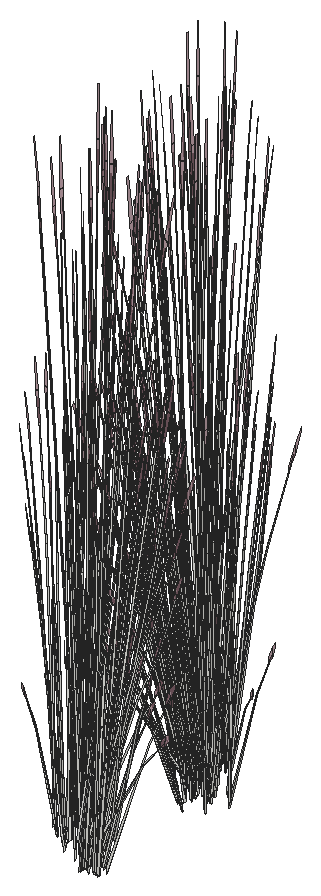
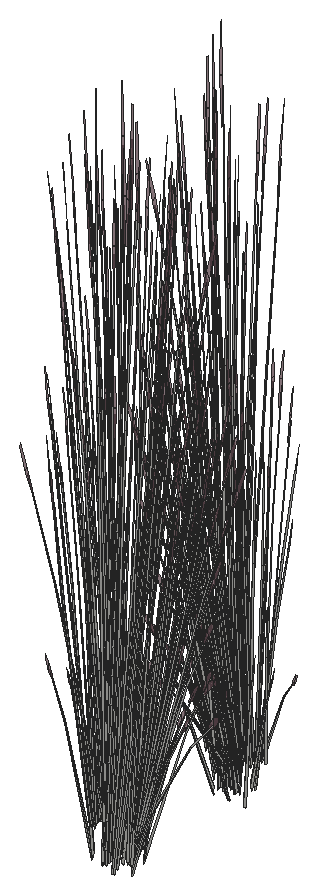
# SketchUp Ruby script. Lengths in inches.
U = 1.inch
M = Sketchup.active_model
def pt(a) = Geom::Point3d.new(a.map { |v| v * U })
def face(e, loops, mat)
  f = e.add_face(loops[0].map { |a| pt(a) })
  loops[1..].each { |l| e.add_face(l.map { |a| pt(a) }).erase! }
  f.material = f.back_material = mat if mat
  f
end
# faces: each face lists its corners as indices into pts; further lists are holes
def faces(e, pts, list, mat = nil) = list.each { |f| face(e, (f[0].is_a?(Array) ? f : [f]).map { |l| l.map { |i| pts[i] } }, mat) }
# xy, xz, yz: faces in a plane at the given z, y or x. An outline is a flat list of corners, or four numbers for a rectangle; further outlines are holes
def ring(l) = l.size == 4 ? [[l[0], l[1]], [l[2], l[1]], [l[2], l[3]], [l[0], l[3]]] : l.each_slice(2).to_a
def flat(e, list, mat, &to3) = list.each { |f| face(e, (f[0].is_a?(Array) ? f : [f]).map { |l| ring(l).map { |u, v| to3.(u, v) } }, mat) }
def xy(e, z, list, mat = nil) = flat(e, list, mat) { |x, y| [x, y, z] }
def xz(e, y, list, mat = nil) = flat(e, list, mat) { |x, z| [x, y, z] }
def yz(e, x, list, mat = nil) = flat(e, list, mat) { |y, z| [x, y, z] }
def lines(e, pts, list) = list.each { |a, b| e.add_line(pt(pts[a]), pt(pts[b])) }
# prism: a flat outline (further loops are holes) pulled along v
def prism(e, loops, v, mat = nil)
  f = face(e, loops, mat); d = Geom::Vector3d.new(v.map { |x| x * U })
  f.pushpull(f.normal.samedirection?(d) ? d.length : -d.length)
end
def box(e, o, s, mat = nil) = prism(e, [[o, [o[0] + s[0], o[1], o[2]], [o[0] + s[0], o[1] + s[1], o[2]], [o[0], o[1] + s[1], o[2]]]], [0, 0, s[2]], mat)
def at(x, y, z, deg = 0) = Geom::Transformation.translation(pt([x, y, z])) * Geom::Transformation.rotation(ORIGIN, Z_AXIS, deg.degrees)
def axes(o, x, y, z) = Geom::Transformation.new([*x, 0, *y, 0, *z, 0, *pt(o).to_a, 1])
def part(name) = M.definitions.add(name)
# library, detail: a bought-in or finely detailed component or shape, given as its bounding box
def library(name, o, s) = part(name).tap { |d| box(d.entities, o, s) }
def detail(e, o, s) = box(e.add_group.entities, o, s)
def put(e, d, t, mat = nil) = e.add_instance(d, t).tap { |i| i.material = mat if mat }
def group(e, t, mat = nil) = e.add_group.tap { |g| g.transformation = t; g.material = mat if mat }.entities
root = M.entities
M.materials.add("LightPink_Translucent").color = [144, 107, 117]
M.materials["LightPink_Translucent"].alpha = 0.75
c1 = part("blade")
p = [[2.15,0.21,22],[0,0.17,0],[0.09,0.45,0],[2.18,0.31,22],[2.29,0.31,22],[0.38,0.45,0],
  [2.48,0.24,33],[2.49,0.24,33],[2.48,0.22,33]]
faces(c1.entities,p,[[0,1,2,3],[4,5,2,3],[6,3,4,7],[8,0,3,6]])
c2 = part("seeds")
p = [[0.3,-0.1,1.38],[-0.01,-0.03,1.59],[-0.01,-0.03,0.03],[0.14,-0.07,-0.07],[0.29,-0.03,3],[0.15,0.01,3.11]]
faces(c2.entities,p,[[0,1,2,3],[1,0,4,5]],"LightPink_Translucent")
c3 = part("blade with seeds")
put(c3.entities,c1,at(0,0,0))
put(c3.entities,c2,axes([2.4,0.25,30.99],[1.5799,-0.05474,1.17369],[-0.12525,1.92788,0.29478],[-0.07173,-0.02425,1.56792]))
put(root,c3,axes([330.45,409.64,1400.48],[0.33032,0.23318,0.49651],[-0.19744,0.41812,0],[-0.07523,-0.05311,1.57504]))
put(root,c3,axes([331.62,408.02,1400.72],[0.17124,-0.42022,0.44739],[0.35581,0.20224,-0.21531],[0,0.09687,1.43643]))
put(root,c3,axes([333.3,409.9,1402.71],[-0.03191,-0.04083,1.77383],[0.06981,-0.43764,-0.16761],[0.12571,-0.02796,0.31391]))
put(root,c3,axes([329.14,408.125,1402.72],[-0.05763,0.06055,1.74944],[0.0049,0.44239,-0.27667],[-0.13211,0.05753,0.14031]))
put(root,c3,axes([331.55,408.26,1400.29],[0,0.53934,-0.05637],[-0.44133,0,0],[0,0.01695,1.79368]))
put(root,c3,axes([329.53,408.07,1402.68],[-0.09562,0.42421,-0.51099],[-0.32782,-0.1454,-0.3958],[-0.13199,0.0389,0.97773]))
put(root,c3,axes([329.51,407.71,1403.03],[0.17758,0.42229,-0.1216],[-0.31518,0.20752,-0.67495],[-0.13282,0.05572,1.02557]))
put(root,c3,axes([331.58,407.88,1400.21],[0.21202,0.39143,-0.44739],[-0.32115,0.27564,0.21531],[0.06861,0.04843,1.43643]))
put(root,c3,axes([333.02,409.54,1401.93],[-0.06755,-0.39203,-0.03492],[0.31928,-0.09013,-0.15832],[0.06667,0.02485,0.52218]))
put(root,c3,axes([330.26,409.88,1400.375],[-0.22066,0.46731,0],[-0.36918,-0.26061,-0.51607],[-0.08408,-0.05936,1.63711]))
put(root,c3,axes([332.19,409.53,1403.03],[0.0189,-0.47427,-0.1216],[0.35781,0.01296,-0.67495],[0.13781,0.03295,1.02557]))
put(root,c3,axes([332.52,408.26,1400.48],[0,-0.46636,0.49651],[0.39487,0,0],[0,0.10622,1.57504]))
put(root,c3,axes([331.53,408.61,1400.72],[0.38326,-0.02879,0.44739],[0.03466,0.47788,-0.21531],[-0.06861,0.04843,1.43643]))
put(root,c3,axes([331.77,408.12,1400.62],[0.32884,-0.136,0.1448],[0.11516,0.38837,-0.41347],[0,0.08547,1.26744]))
put(root,c3,axes([332.14,409.34,1403.05],[-0.20082,-0.29199,0.35414],[0.2293,-0.2764,-0.4572],[0.1165,0.04206,0.87481]))
put(root,c3,axes([331.1875,408.84,1400.21],[-0.38326,0.02879,-0.44739],[-0.03466,-0.47788,0.21531],[-0.06861,0.04843,1.43643]))
put(root,c3,axes([332.99,409.07,1400.59],[-0.085,-0.1147,1.43002],[0.1106,-0.37943,-0.30754],[0.17198,0.0514,0.61141]))
put(root,c3,axes([331.47,409.48,1400.2],[0.35581,0.20937,0],[-0.17124,0.43505,0],[0,0,1.74954]))
put(root,c3,axes([332.5,409.24,1402.72],[0.07571,-0.00789,1.74944],[0.20767,-0.36231,-0.27667],[0.13467,0.04783,0.14031]))
put(root,c3,axes([331.61,409.95,1400.19],[-0.21791,-0.46895,-0.05142],[0.36918,-0.26061,0.51607],[-0.09097,0.04465,1.6363]))
put(root,c3,axes([331.53,408.8125,1400.62],[0.26075,0.2802,0.1448],[-0.2175,0.31612,-0.41347],[-0.06054,0.04274,1.26744]))
put(root,c3,axes([329.47,408.89,1402.73],[-0.08753,-0.42921,0.48003],[0.34336,-0.07449,0.3958],[-0.1012,0.10094,0.9933]))
put(root,c3,axes([329.41,408.8,1402.73],[-0.2423,-0.19613,0.0643],[0.14107,-0.2793,0.50621],[-0.07768,0.0903,0.77189]))
put(root,c3,axes([329.52,408.29,1401.875],[0.12246,-0.09864,1.71376],[0.1031,0.45582,0.13857],[-0.19225,0.10302,0.73262]))
put(root,c3,axes([332.21,409.3,1402.98],[0.35281,0.01123,-0.71045],[-0.0237,0.47284,0.08574],[0.14947,0.0499,1.00501]))
put(root,c3,axes([331.8125,409.68,1400.48],[0.33032,-0.23318,0.49651],[0.19744,0.41812,0],[-0.07523,0.05311,1.57504]))
put(root,c3,axes([331.34,409.31,1400.29],[0.15345,0.53576,-0.06012],[-0.43845,0.18773,0],[0.00536,0.01871,1.72173]))
put(root,c3,axes([331.51,409.89,1400.03],[-0.32928,-0.11539,-0.30978],[0.08291,-0.40636,0.30978],[-0.06638,0.04686,1.38974]))
put(root,c3,axes([329.14,409.0625,1400.59],[0.12266,0.03828,1.43002],[0.07906,0.39104,-0.30754],[-0.16661,0.0732,0.61141]))
put(root,c3,axes([329.6875,408.74,1403.05],[0.30722,-0.06665,0.35414],[0.08112,0.381,-0.4572],[-0.08804,0.10234,0.87481]))
put(root,c3,axes([332.78,408.34,1400.375],[0.44133,0,0],[0,0.52122,-0.51607],[0,0.11871,1.63711]))
put(root,c3,axes([328.5,408.57,1402.71],[0.04504,0.01251,1.77383],[0.13934,0.41205,-0.16761],[-0.0922,0.10815,0.31391]))
put(root,c3,axes([332.61,408.61,1400.2],[-0.44111,-0.00373,-0.04976],[0,-0.52122,0.49943],[-0.01386,0.11865,1.58352]))
put(root,c3,axes([331.65,408.15,1400.67],[0.39748,0.22252,-0.29095],[-0.19139,0.46966,-0.50002],[0.01249,0.11531,1.59708]))
put(root,c3,axes([328.88,409.88,1400.77],[0.14709,-0.21136,1.1486],[0.05804,0.3346,0.84392],[-0.1063,0.05991,0.25299]))
put(root,c3,axes([332.42,409.49,1402.53],[0.20082,0.29199,-0.35414],[-0.2293,0.2764,0.4572],[0.1165,0.04206,0.87481]))
put(root,c3,axes([332.52,408.68,1400.03],[-0.24637,0.29097,-0.30978],[-0.24637,-0.29097,0.30978],[0,0.09372,1.38974]))
put(root,c3,axes([331.46,408.71,1400.67],[0.04113,0.53214,-0.29095],[-0.42835,0.03218,-0.50002],[-0.07543,0.07088,1.59708]))
put(root,c3,axes([332.32,409.6,1402.73],[-0.01777,0.35463,0.0643],[-0.26836,-0.00972,0.50621],[0.1028,0.03711,0.77189]))
put(root,c3,axes([331.61,408.5,1400.21],[-0.17124,0.42022,-0.44739],[-0.35581,-0.20224,0.21531],[0,0.09687,1.43643]))
put(root,c3,axes([329.43,408.97,1402.53],[-0.30722,0.06665,-0.35414],[-0.08112,-0.381,0.4572],[-0.08804,0.10234,0.87481]))
put(root,c3,axes([332.34,409.49,1402.73],[-0.26024,0.30729,0.48003],[-0.22444,-0.32634,0.3958],[0.1221,0.05668,0.9933]))
put(root,c3,axes([328.99,409.83,1403.65],[0.31145,0.12449,-0.06488],[-0.0958,0.38314,-0.29416],[-0.05094,0.05817,0.97024]))
put(root,c3,axes([331.2,409.12,1400.06],[-0.23773,0.35053,-0.62353],[-0.29532,-0.31785,-0.16365],[-0.09526,0.08744,1.37633]))
put(root,c3,axes([331.52,409.85,1403.05],[-0.05451,-0.37564,0.35414],[0.31161,-0.09919,-0.4572],[0.0837,0.10765,0.87481]))
put(root,c3,axes([331.62,409.71,1400.33],[0.44186,0.15158,0.30756],[-0.11054,0.54181,-0.36492],[-0.07313,0.06781,1.64885]))
put(root,c3,axes([331.59,410.07,1400.02],[-0.33032,0.23318,-0.49651],[-0.19744,-0.41812,0],[-0.07523,0.05311,1.57504]))
put(root,c3,axes([332.6875,408.69,1400.02],[0,0.46636,-0.49651],[-0.39487,0,0],[0,0.10622,1.57504]))
put(root,c3,axes([331.7,408.74,1401.875],[-0.1311,-0.08035,1.71376],[0.27131,-0.33708,0.13857],[0.16909,0.15206,0.73262]))
put(root,c3,axes([331.72,407.6875,1402.47],[-0.30498,-0.24231,1.38283],[0.32203,-0.37727,0.59665],[0.0984,0.22736,1.33663]))
put(root,c3,axes([329.53,408.71,1403.03],[0.32648,0.25715,-0.1216],[-0.18809,0.3724,-0.67495],[-0.09224,0.12945,1.02557]))
put(root,c3,axes([332.18,409.66,1400.77],[-0.19872,-0.13409,1.1486],[0.2566,-0.13625,0.84392],[0.06921,0.11541,0.25299]))
put(root,c3,axes([331.49,410.04,1403.03],[0.21031,-0.39918,-0.1216],[0.30457,0.22997,-0.67495],[0.10587,0.11278,1.02557]))
put(root,c3,axes([329.97,408.59,1401.875],[0.08815,-0.14329,1.71376],[0.22258,0.38678,0.13857],[-0.15267,0.17614,0.73262]))
put(root,c3,axes([329.6875,409.01,1402.68],[0.09067,0.42583,-0.51099],[-0.34336,0.07449,-0.3958],[-0.0984,0.11438,0.97773]))
put(root,c3,axes([330.1,409.5,1403.05],[0.23881,-0.24554,0.35414],[0.22606,0.28036,-0.4572],[-0.0344,0.14245,0.87481]))
put(root,c3,axes([331.89,410,1400.375],[0.22066,0.46731,0],[-0.36918,0.26061,-0.51607],[-0.08408,0.05936,1.63711]))
put(root,c3,axes([331.21,410.37,1402.71],[0.00104,-0.05646,1.77383],[0.30246,-0.2491,-0.16761],[0.10506,0.08891,0.31391]))
put(root,c3,axes([332.24,410.16,1399.49],[0.02571,-0.06733,1.76342],[0.32373,-0.19829,-0.26939],[0.09815,0.10263,0.30037]))
put(root,c3,axes([331.7,408.15,1400.84],[-0.00964,-0.43909,1.41272],[0.43635,0.11382,0.59816],[-0.1032,0.24027,1.3335]))
put(root,c3,axes([331.8125,408.63,1400.09],[0.12941,0.42699,-0.69212],[-0.37279,0.15378,-0.18165],[0.0143,0.14459,1.52773]))
put(root,c3,axes([329.88,409.73,1402.73],[-0.29004,-0.02173,0.0643],[0.00795,-0.32812,0.50621],[-0.03035,0.12569,0.77189]))
put(root,c3,axes([329.27,410.1,1399.49],[0.04734,0.04659,1.76342],[0.08027,0.4317,-0.26939],[-0.10492,0.09206,0.30037]))
put(root,c3,axes([329.98,409.76,1402.73],[-0.25132,-0.3182,0.48003],[0.2669,-0.27442,0.3958],[-0.04636,0.14929,0.9933]))
put(root,c3,axes([331.74,409.84,1402.68],[0.34827,-0.11086,-0.51099],[0.06092,0.41983,-0.3958],[0.09354,0.12031,0.97773]))
put(root,c3,axes([330.77,409.91,1403.05],[0.1064,-0.35863,0.35414],[0.31043,0.1046,-0.4572],[0.02846,0.14439,0.87481]))
put(root,c3,axes([332.22,410.27,1400.67],[-0.22633,-0.01463,1.0506],[0.14947,-0.31064,0.58006],[0.08941,0.11036,0.8241]))
put(root,c3,axes([331.56,410.1875,1402.73],[-0.16041,0.29625,0.0643],[-0.22843,-0.17248,0.50621],[0.07385,0.09498,0.77189]))
put(root,c3,axes([331.1875,411.1875,1403.65],[0.2439,-0.26754,-0.06488],[0.22348,0.29302,-0.29416],[0.01573,0.08303,0.97024]))
put(root,c3,axes([331.63,410.1,1402.73],[-0.35104,0.10702,0.48003],[-0.06092,-0.41983,0.3958],[0.08256,0.12373,0.9933]))
put(root,c3,axes([329.9,408.95,1401.875],[0.06572,-0.16029,1.71376],[0.27569,0.33172,0.13857],[-0.12437,0.20675,0.73262]))
put(root,c3,axes([331.48,409.52,1400.59],[0.00623,-0.15459,1.43002],[0.29764,-0.17268,-0.30754],[0.09188,0.18503,0.61141]))
put(root,c3,axes([330.67,410.23,1402.73],[-0.26007,0.1585,0.0643],[-0.12729,-0.28902,0.50621],[0.02512,0.1274,0.77189]))
put(root,c3,axes([329.98,409.85,1402.53],[-0.23881,0.24554,-0.35414],[-0.22606,-0.28036,0.4572],[-0.0344,0.14245,0.87481]))
put(root,c3,axes([329.15,409.78,1402.72],[-0.00877,0.09229,1.74944],[0.24897,0.32105,-0.27667],[-0.06518,0.15182,0.14031]))
put(root,c3,axes([329.95,409.57,1403.4],[0.3879,0.02311,-0.13498],[-0.0106,0.43749,-0.74919],[-0.02694,0.1685,1.13838]))
put(root,c3,axes([330.67,410.06,1403.03],[0.34538,-0.21713,-0.1216],[0.16972,0.38536,-0.67495],[0.04557,0.16239,1.02557]))
put(root,c3,axes([330.77,410.2,1403.0625],[-0.34777,-0.12192,0.53283],[0.11892,-0.40083,0.43934],[0.0209,0.15763,1.10256]))
put(root,c3,axes([330.13,410.8,1400.77],[-0.00913,-0.2773,1.1486],[0.22824,0.19778,0.84392],[-0.04489,0.13217,0.25299]))
put(root,c3,axes([330.73,410.14,1399.49],[0.05712,-0.02538,1.76342],[0.34359,0.13968,-0.26939],[0.01005,0.15742,0.30037]))
put(root,c3,axes([330.21,409.73,1403],[0.25266,0.31335,-0.5672],[-0.2669,0.27442,-0.43934],[-0.03844,0.15921,1.08528]))
put(root,c3,axes([329.9375,410.21,1400.82],[0.32063,-0.08258,0.06507],[0.07371,0.33271,-0.86304],[-0.02033,0.16842,0.7736]))
put(root,c3,axes([330.96,410.04,1402.68],[0.34695,0.11691,-0.51099],[-0.11892,0.40083,-0.3958],[0.03181,0.16138,0.97773]))
put(root,c3,axes([331.16,409.21,1401.875],[-0.08068,-0.14973,1.71376],[0.3728,-0.12606,0.13857],[0.08426,0.23506,0.73262]))
put(root,c3,axes([330.8,410.28,1402.53],[-0.1064,0.35863,-0.35414],[-0.31043,-0.1046,0.4572],[0.02846,0.14439,0.87481]))
put(root,c3,axes([330.13,409.59,1403.34],[-0.00918,0.43138,-0.7886],[-0.38672,-0.02897,0.09517],[-0.04081,0.18275,1.11556]))
put(root,c3,axes([329.125,410.72,1402.71],[0.04004,-0.02816,1.77383],[0.33095,0.18728,-0.16761],[-0.00778,0.15594,0.31391]))
put(root,c3,axes([330.5,409.29,1401.875],[-0.00864,-0.17899,1.71376],[0.37441,0.11874,0.13857],[-0.02316,0.25508,0.73262]))
put(root,c3,axes([330.84,409.96,1402.98],[0.16845,0.3792,-0.71045],[-0.34676,0.21133,0.08574],[0.03939,0.18322,1.00501]))
put(root,c3,axes([329.86,410.56,1400.59],[0.11138,-0.07357,1.43002],[0.27499,0.22183,-0.30754],[-0.08185,0.19194,0.61141]))
put(root,c3,axes([330.58,410.92,1402.72],[0.04474,0.0751,1.74944],[0.36104,0.0295,-0.27667],[0.03631,0.16562,0.14031]))
put(root,c3,axes([330.01,410.2,1401.36],[0.00775,-0.24075,1.54345],[0.34877,0.12716,0.21329],[-0.03022,0.25658,0.72882]))
put(root,c3,axes([330.27,421.53,1401.875],[0.08068,0.14973,1.71376],[-0.3728,0.12606,0.13857],[-0.08426,-0.23506,0.73262]))
put(root,c3,axes([330.89,420.54,1402.72],[-0.05398,-0.06539,1.74944],[-0.36026,0.04145,-0.27667],[-0.0575,-0.15639,0.14031]))
put(root,c3,axes([331.72,421.32,1400.59],[-0.10032,0.0944,1.43002],[-0.30046,-0.16522,-0.30754],[0.05569,-0.20547,0.61141]))
put(root,c3,axes([331.27,421.64,1402.98],[-0.16845,-0.3792,-0.71045],[0.34676,-0.21133,0.08574],[-0.03939,-0.18322,1.00501]))
put(root,c3,axes([330.17,421.14,1400.59],[-0.02137,0.15256,1.43002],[-0.31245,0.12771,-0.30754],[-0.07303,-0.19719,0.61141]))
put(root,c3,axes([330.98,420.8,1399.49],[-0.0592,0.0168,1.76342],[-0.32738,-0.18913,-0.26939],[0.00549,-0.15776,0.30037]))
put(root,c3,axes([331.97,422.01,1402.98],[0.00918,-0.43138,-0.71045],[0.38672,0.02897,0.08574],[0.04081,-0.18275,1.00501]))
put(root,c3,axes([332.51,421.34,1402.72],[-0.00341,-0.09282,1.74944],[-0.28775,-0.26825,-0.27667],[0.04449,-0.16261,0.14031]))
put(root,c3,axes([331.3,421.32,1402.53],[0.1064,-0.35863,-0.35414],[0.31043,0.1046,0.4572],[-0.02846,-0.14439,0.87481]))
put(root,c3,axes([331.53,421.8,1401.875],[-0.06572,0.16029,1.71376],[-0.27569,-0.33172,0.13857],[0.12437,-0.20675,0.73262]))
put(root,c3,axes([332.43,421.01,1402.71],[-0.03584,0.03562,1.77383],[-0.35118,-0.12018,-0.16761],[-0.01271,-0.15545,0.31391]))
put(root,c3,axes([331.14,421.57,1402.68],[-0.34695,-0.11691,-0.51099],[0.11892,-0.40083,-0.3958],[-0.03181,-0.16138,0.97773]))
put(root,c3,axes([331.35,420.5625,1400.77],[0.04528,0.27194,1.1486],[-0.25117,-0.15062,0.84392],[0.02703,-0.13924,0.25299]))
put(root,c3,axes([331.89,421.87,1402.68],[-0.25266,-0.31335,-0.51099],[0.2669,-0.27442,-0.3958],[0.03844,-0.15921,0.97773]))
put(root,c3,axes([330.52,420.33,1402.71],[-0.00658,0.0559,1.77383],[-0.32474,0.20287,-0.16761],[-0.09556,-0.1037,0.31391]))
put(root,c3,axes([330.45,421.32,1403.09],[0.39316,-0.11987,0.53763],[0.06823,0.47021,0.4433],[-0.09247,-0.13858,1.11249]))
put(root,c3,axes([331.34,421.4,1402.73],[0.34777,0.12192,0.48003],[-0.11892,0.40083,0.3958],[-0.0209,-0.15763,0.9933]))
put(root,c3,axes([331.4375,421.55,1403.03],[-0.34538,0.21713,-0.1216],[-0.16972,-0.38536,-0.67495],[-0.04557,-0.16239,1.02557]))
put(root,c3,axes([332.15,422.04,1403.03],[-0.3879,-0.02311,-0.1216],[0.0106,-0.43749,-0.67495],[0.02694,-0.1685,1.02557]))
put(root,c3,axes([332.13,421.76,1402.53],[0.23881,-0.24554,-0.35414],[0.22606,0.28036,0.4572],[0.0344,-0.14245,0.87481]))
put(root,c3,axes([330.0625,420.89,1400.77],[0.18411,0.16231,1.1486],[-0.26813,0.09757,0.84392],[-0.05737,-0.12474,0.25299]))
put(root,c3,axes([331.43,421.375,1402.73],[0.26007,-0.1585,0.0643],[0.12729,0.28902,0.50621],[-0.02512,-0.1274,0.77189]))
put(root,c3,axes([330.51,421.75,1402.98],[-0.30095,-0.22541,-0.71045],[0.21388,-0.395,0.08574],[-0.10904,-0.13459,1.00501]))
put(root,c3,axes([330.4,421.45,1402.53],[-0.05451,-0.37564,-0.35414],[0.31161,-0.09919,0.4572],[-0.0837,-0.10765,0.87481]))
put(root,c3,axes([330.54,421.42,1402.73],[0.16041,-0.29625,0.0643],[0.22843,0.17248,0.50621],[-0.07385,-0.09498,0.77189]))
put(root,c3,axes([329.92,421.38,1399.49],[-0.03419,0.06144,1.76342],[-0.3455,0.13246,-0.26939],[-0.08346,-0.12049,0.30037]))
put(root,c3,axes([330.49,423.07,1400.1],[-0.14494,-0.47823,-0.69835],[0.41752,-0.17223,-0.18329],[-0.01602,-0.16194,1.54149]))
put(root,c3,axes([329.73,422,1401.875],[0.1311,0.08035,1.71376],[-0.27131,0.33708,0.13857],[-0.16909,-0.15206,0.73262]))
put(root,c3,axes([332.43,421.61,1399.49],[-0.05283,-0.03674,1.76342],[-0.13569,-0.41045,-0.26939],[0.09154,-0.11138,0.30037]))
put(root,c3,axes([331.33,421.7,1403.05],[-0.1064,0.35863,0.35414],[-0.31043,-0.1046,-0.4572],[-0.02846,-0.14439,0.87481]))
put(root,c3,axes([330.37,421.76,1402.68],[-0.34827,0.11086,-0.51099],[-0.06092,-0.41983,-0.3958],[-0.09354,-0.12031,0.97773]))
put(root,c3,axes([332.125,421.85,1402.73],[0.25132,0.3182,0.48003],[-0.2669,0.27442,0.3958],[0.04636,-0.14929,0.9933]))
put(root,c3,axes([330.61,421.39,1403.43],[-0.23555,0.44708,-0.13619],[-0.34112,-0.25757,-0.75594],[-0.11858,-0.12631,1.14864]))
put(root,c3,axes([332.22,421.88,1402.73],[0.29004,0.02173,0.0643],[-0.00795,0.32812,0.50621],[0.03035,-0.12569,0.77189]))
put(root,c3,axes([332,422.1,1403.05],[-0.23881,0.24554,0.35414],[-0.22606,-0.28036,-0.4572],[0.0344,-0.14245,0.87481]))
put(root,c3,axes([332.42,422.76,1402.98],[0.18436,-0.36797,-0.71045],[0.32306,0.26151,0.08574],[0.11008,-0.13332,1.00501]))
put(root,c3,axes([330.43,421.69,1400.375],[-0.22066,-0.46731,0],[0.36918,-0.26061,-0.51607],[0.08408,-0.05936,1.63711]))
put(root,c3,axes([332.41,422.59,1402.68],[-0.09067,-0.42583,-0.51099],[0.34336,-0.07449,-0.3958],[0.0984,-0.11438,0.97773]))
put(root,c3,axes([330.92,421.13,1400.13],[-0.2439,0.26754,-0.03893],[-0.22348,-0.29302,-0.17649],[-0.01573,-0.08303,0.58215]))
put(root,c3,axes([329.71,421.26,1402.72],[-0.07594,-0.00329,1.74944],[-0.24177,0.32918,-0.27667],[-0.129,-0.06726,0.14031]))
put(root,c3,axes([332.58,422.9,1403.03],[-0.32648,-0.25715,-0.1216],[0.18809,-0.3724,-0.67495],[0.09224,-0.12945,1.02557]))
put(root,c3,axes([331.23,424.3,1401.33],[0.305,0.18805,1.51261],[-0.29879,0.40513,0.59816],[-0.13384,-0.24012,1.26806]))
put(root,c3,axes([330.59,421.76,1403.05],[0.05451,0.37564,0.35414],[-0.31161,0.09919,-0.4572],[-0.0837,-0.10765,0.87481]))
put(root,c3,axes([329.63,423,1400.02],[0,-0.46636,-0.49651],[0.39487,0,0],[0,-0.10622,1.57504]))
put(root,c3,axes([330.73,421.62,1400.02],[0.33032,-0.23318,-0.49651],[0.19744,0.41812,0],[0.07523,-0.05311,1.57504]))
put(root,c3,axes([332.69,422.43,1400.59],[-0.12609,-0.01381,1.43002],[-0.12917,-0.37055,-0.30754],[0.1549,-0.10482,0.61141]))
put(root,c3,axes([329.65,422,1403.09],[0.29147,-0.34417,0.53763],[0.25138,0.3655,0.4433],[-0.13675,-0.06349,1.11249]))
put(root,c3,axes([333.38,422.79,1402.71],[-0.0461,-0.00354,1.77383],[-0.19143,-0.37951,-0.16761],[0.07688,-0.12478,0.31391]))
put(root,c3,axes([331.12,422.58,1400.06],[0.23773,-0.35053,-0.62353],[0.29532,0.31785,-0.16365],[0.09526,-0.08744,1.37633]))
put(root,c3,axes([332.84,421.75,1400.77],[-0.11756,0.2374,1.1486],[-0.10105,-0.31895,0.84392],[0.09709,-0.07992,0.25299]))
put(root,c3,axes([332.67,422.64,1402.53],[0.30722,-0.06665,-0.35414],[0.08112,0.381,0.4572],[0.08804,-0.10234,0.87481]))
put(root,c3,axes([329.78,422,1402.73],[0.01777,-0.35463,0.0643],[0.26836,0.00972,0.50621],[-0.1028,-0.03711,0.77189]))
put(root,c3,axes([330.71,423.19,1400.21],[0.17124,-0.42022,-0.44739],[0.35581,0.20224,0.21531],[0,-0.09687,1.43643]))
put(root,c3,axes([329.68,422.11,1402.53],[-0.20082,-0.29199,-0.35414],[0.2293,-0.2764,0.4572],[-0.1165,-0.04206,0.87481]))
put(root,c3,axes([330.86,422.98,1400.67],[-0.04113,-0.53214,-0.29095],[0.42835,-0.03218,-0.50002],[0.07543,-0.07088,1.59708]))
put(root,c3,axes([329.8,423.01,1400.03],[0.24637,-0.29097,-0.30978],[0.24637,0.29097,0.30978],[0,-0.09372,1.38974]))
put(root,c3,axes([329.7,421.62,1400.13],[-0.10181,0.3808,-0.03893],[-0.31336,-0.11714,-0.17649],[-0.04758,-0.06228,0.58215]))
put(root,c3,axes([332.42,422.86,1403.05],[-0.30722,0.06665,0.35414],[-0.08112,-0.381,-0.4572],[0.08804,-0.10234,0.87481]))
put(root,c3,axes([330.67,423.54,1400.67],[-0.39748,-0.22252,-0.29095],[0.19139,-0.46966,-0.50002],[-0.01249,-0.11531,1.59708]))
put(root,c3,axes([329.53,423.36,1400.375],[-0.44133,0,0],[0,-0.52122,-0.51607],[0,-0.11871,1.63711]))
put(root,c3,axes([329.61,422.42,1400.59],[0.06891,0.12984,1.43002],[-0.15879,0.35293,-0.30754],[-0.16304,-0.08436,0.61141]))
put(root,c3,axes([330.81,421.81,1400.03],[0.32928,0.11539,-0.30978],[-0.08291,0.40636,0.30978],[0.06638,-0.04686,1.38974]))
put(root,c3,axes([329.89,422.31,1402.98],[-0.35281,-0.01123,-0.71045],[0.0237,-0.47284,0.08574],[-0.14947,-0.0499,1.00501]))
put(root,c3,axes([332.7,422.8,1402.73],[0.2423,0.19613,0.0643],[-0.14107,0.2793,0.50621],[0.07768,-0.0903,0.77189]))
put(root,c3,axes([332.63,422.72,1402.73],[0.08753,0.42921,0.48003],[-0.34336,0.07449,0.3958],[0.1012,-0.10094,0.9933]))
put(root,c3,axes([333.55,423.24,1402.72],[0.04898,-0.07104,1.74944],[-0.06269,-0.43574,-0.27667],[0.12289,-0.08262,0.14031]))
put(root,c3,axes([329.875,423.22,1400.33],[-0.32829,0.39208,0.30756],[-0.32849,-0.38796,-0.36492],[-0.01146,-0.11134,1.64885]))
put(root,c3,axes([329.42,421.54,1402.71],[0.02617,0.04654,1.77383],[-0.12614,0.41836,-0.16761],[-0.12775,0.00303,0.31391]))
put(root,c3,axes([330.92,423.4,1400.43],[0.39767,0.22603,0.24065],[-0.19139,0.46966,0.50002],[0,-0.10827,1.60543]))
put(root,c3,axes([330.77,424.04,1400.4375],[0.09355,-0.55261,-0.23429],[0.44354,0.09633,0.51271],[-0.0775,-0.07631,1.5644]))
put(root,c3,axes([329.78,422.4,1402.68],[-0.25628,0.30892,-0.51099],[-0.22444,-0.32634,-0.3958],[-0.13021,-0.047,0.97773]))
put(root,c3,axes([329.97,422.27,1403.05],[0.20082,0.29199,0.35414],[-0.2293,0.2764,-0.4572],[-0.1165,-0.04206,0.87481]))
put(root,c3,axes([329.2,422.8125,1400.77],[0.22533,-0.03337,1.1486],[-0.14293,0.29403,0.84392],[-0.11135,-0.04411,0.25299]))
put(root,c3,axes([330.79,423.09,1400.72],[-0.38326,0.02879,0.44739],[-0.03466,-0.47788,-0.21531],[0.06861,-0.04843,1.43643]))
put(root,c3,axes([329.91,422.08,1403.03],[-0.0189,0.47427,-0.1216],[-0.35781,-0.01296,-0.67495],[-0.13781,-0.03295,1.02557]))
put(root,c3,axes([329.8,423.43,1400.48],[0,0.46636,0.49651],[-0.39487,0,0],[0,-0.10622,1.57504]))
put(root,c3,axes([332.59,423.9,1403.03],[-0.17758,-0.42229,-0.1216],[0.31518,-0.20752,-0.67495],[0.13282,-0.05572,1.02557]))
put(root,c3,axes([332.57,423.54,1402.68],[0.09562,-0.42421,-0.51099],[0.32782,0.1454,-0.3958],[0.13199,-0.0389,0.97773]))
put(root,c3,axes([332.06,421.8125,1400.375],[0.22066,-0.46731,0],[0.36918,0.26061,-0.51607],[0.08408,0.05936,1.63711]))
put(root,c3,axes([329.46,422.73,1401.875],[0.14639,-0.01056,1.71376],[-0.09712,0.45778,0.13857],[-0.20862,-0.02831,0.73262]))
put(root,c3,axes([330.73,423.8125,1400.21],[-0.21202,-0.39143,-0.44739],[0.32115,-0.27564,0.21531],[-0.06861,-0.04843,1.43643]))
put(root,c3,axes([330.78,423.26,1400.36],[0.15345,0.52148,0.45755],[-0.43845,0.18134,0.17955],[0.00536,-0.09582,1.58856]))
put(root,c3,axes([332.92,423.66,1399.98],[-0.22732,0.05597,1.41583],[-0.03618,-0.44548,0.08104],[0.15921,-0.06743,0.80566]))
put(root,c3,axes([333.34,423.26,1400.26],[-0.21881,-0.29821,-0.06488],[0.23965,-0.27324,-0.29416],[0.0679,-0.01924,0.97024]))
put(root,c3,axes([330.7,423.67,1400.72],[-0.17124,0.42022,0.44739],[-0.35581,-0.20224,-0.21531],[0,-0.09687,1.43643]))
put(root,c3,axes([331.33,423.3,1400.21],[0,-0.53961,0],[0.44133,0,0],[0,0,1.79456]))
put(root,c3,axes([331.87,422.06,1400.48],[-0.33032,-0.23318,0.49651],[0.19744,-0.41812,0],[0.07523,0.05311,1.57504]))
put(root,c3,axes([332.51,423.69,1402.98],[0.31014,-0.20596,-0.71045],[0.17284,0.42397,0.08574],[0.14985,-0.04816,1.00501]))
put(root,c3,axes([330.54,423.96,1400.06],[-0.36714,-0.07646,-0.62353],[0.07747,-0.47163,-0.16365],[-0.10956,-0.05715,1.37633]))
put(root,c3,axes([331.12,422.96,1400.36],[-0.29264,0.42323,0.45755],[-0.34767,-0.3736,0.17955],[0.07055,-0.04224,1.58856]))
put(root,c3,axes([331.44,423.72,1400.3],[-0.32829,-0.4014,-0.06131],[0.32849,-0.40164,0],[-0.01146,-0.01402,1.75571]))
put(root,c3,axes([330.61,422.27,1400.47],[-0.10196,0.46348,0.17642],[-0.3731,-0.13116,0.35086],[0.06445,-0.00226,1.60407]))
put(root,c3,axes([332.47,423.77,1403.05],[-0.29332,-0.1301,0.35414],[0.08555,-0.37955,-0.4572],[0.11809,-0.0348,0.87481]))
put(root,c3,axes([329.4,423.08,1402.73],[0.09971,-0.42522,0.48003],[0.32782,0.1454,0.3958],[-0.12892,0.02555,0.9933]))
put(root,c3,axes([330.46,422.64,1399.59],[-0.3474,0.18671,1.28929],[-0.11057,-0.53572,0.50096],[0.21332,0.00891,1.46642]))
put(root,c3,axes([331.39,422.78,1400.62],[0.06809,-0.4162,0.1448],[0.33266,0.07225,-0.41347],[0.06054,0.04274,1.26744]))
put(root,c3,axes([329.37,422.97,1402.73],[-0.12963,-0.31798,0.0643],[0.23638,-0.15564,0.50621],[-0.1042,0.03071,0.77189]))
put(root,c3,axes([330.82,423.77,1400.36],[0.44609,0.09826,0.45755],[-0.09078,0.55493,0.17955],[-0.06519,-0.05359,1.58856]))
put(root,c3,axes([333.17,423.37,1399.49],[-0.01845,-0.0708,1.76342],[0.12793,-0.41416,-0.26939],[0.12905,-0.00596,0.30037]))
put(root,c3,axes([329.36,423.29,1399.49],[0.00895,0.0735,1.76342],[-0.18044,0.38382,-0.26939],[-0.12817,-0.01935,0.30037]))
put(root,c3,axes([331.25,422.89,1400.72],[-0.21202,-0.39143,0.44739],[0.32115,-0.27564,-0.21531],[0.06861,0.04843,1.43643]))
put(root,c3,axes([330.15,424.68,1400.03],[-0.08291,-0.40636,-0.30978],[0.32928,-0.11539,0.30978],[-0.06638,-0.04686,1.38974]))
put(root,c3,axes([330.58,424.66,1400.47],[0.37926,-0.12378,0.17642],[0.09365,0.46065,0.35086],[-0.03382,-0.06712,1.60407]))
put(root,c3,axes([331.36,422.92,1400.67],[0.35635,-0.30962,-0.29095],[0.23697,0.43749,-0.50002],[0.08792,0.04443,1.59708]))
put(root,c3,axes([332.78,423.73,1402.53],[0.29332,0.1301,-0.35414],[-0.08555,0.37955,0.4572],[0.11809,-0.0348,0.87481]))
put(root,c3,axes([330.0625,424.85,1400.02],[-0.33032,-0.23318,-0.49651],[0.19744,-0.41812,0],[-0.07523,-0.05311,1.57504]))
put(root,c3,axes([332.26,422.09,1400.02],[0.33032,0.23318,-0.49651],[-0.19744,0.41812,0],[0.07523,0.05311,1.57504]))
put(root,c3,axes([329.33,423.13,1402.53],[-0.29332,-0.1301,-0.35414],[0.08555,-0.37955,0.4572],[-0.11809,0.0348,0.87481]))
put(root,c3,axes([331.63,423.42,1400.21],[0.39487,0,0],[0,0.48281,0],[0,0,1.78407]))
put(root,c3,axes([330.96,424.03,1400.67],[-0.35635,0.30962,-0.29095],[-0.23697,-0.43749,-0.50002],[-0.08792,-0.04443,1.59708]))
put(root,c3,axes([331.74,422.29,1400.47],[-0.37926,0.12378,0.17642],[-0.09365,-0.46065,0.35086],[0.03382,0.06712,1.60407]))
put(root,c3,axes([331.98,423.26,1401.875],[-0.14639,0.01056,1.71376],[0.09712,-0.45778,0.13857],[0.20862,0.02831,0.73262]))
put(root,c3,axes([332.17,422.27,1400.03],[0.08291,0.40636,-0.30978],[-0.32928,0.11539,0.30978],[0.06638,0.04686,1.38974]))
put(root,c3,axes([332.73,423.89,1402.73],[0.12963,0.31798,0.0643],[-0.23638,0.15564,0.50621],[0.1042,-0.03071,0.77189]))
put(root,c3,axes([331.5,423.18,1400.38],[-0.44609,-0.09826,0.49198],[0.09078,-0.55493,0.19306],[0.06519,0.05359,1.70813]))
put(root,c3,axes([332.71,423.78,1402.73],[-0.09971,0.42522,0.48003],[-0.32782,-0.1454,0.3958],[0.12892,-0.02555,0.9933]))
put(root,c3,axes([331.15,424.55,1400.2],[-0.11516,-0.40207,0],[0.32884,-0.1408,0],[0,0,1.54371]))
put(root,c3,axes([330.93,424.17,1400.62],[-0.06809,0.4162,0.1448],[-0.33266,-0.07225,-0.41347],[-0.06054,-0.04274,1.26744]))
put(root,c3,axes([329.64,423.09,1403.05],[0.29332,0.1301,0.35414],[-0.08555,0.37955,-0.4572],[-0.11809,0.0348,0.87481]))
